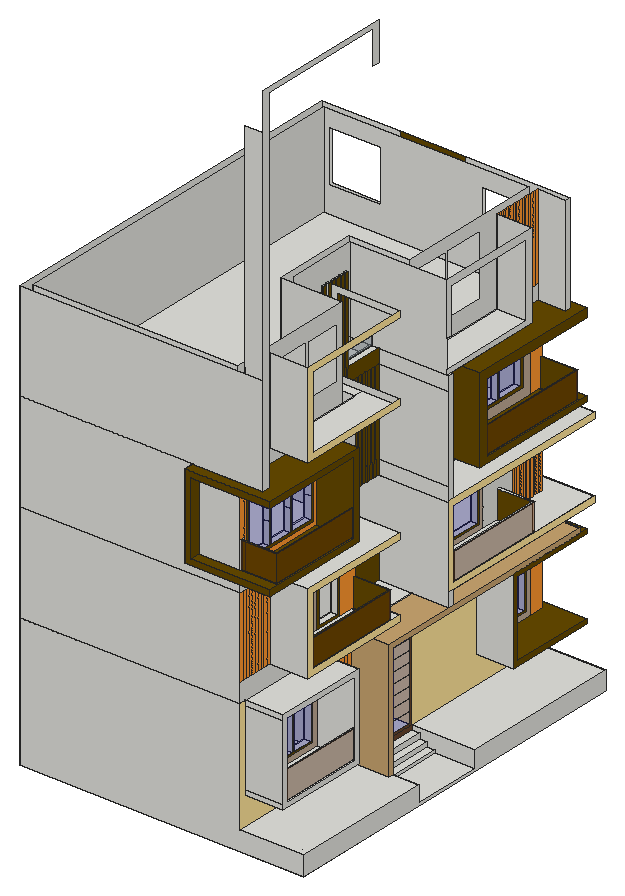
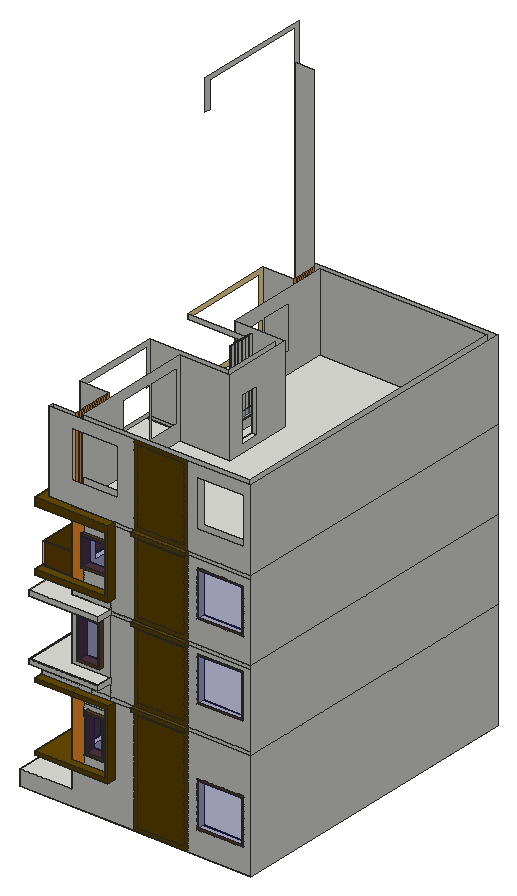
# SketchUp Ruby script. Lengths in inches.
U = 1.inch
M = Sketchup.active_model
def pt(a) = Geom::Point3d.new(a.map { |v| v * U })
def face(e, loops, mat)
  f = e.add_face(loops[0].map { |a| pt(a) })
  loops[1..].each { |l| e.add_face(l.map { |a| pt(a) }).erase! }
  f.material = f.back_material = mat if mat
  f
end
# faces: each face lists its corners as indices into pts; further lists are holes
def faces(e, pts, list, mat = nil) = list.each { |f| face(e, (f[0].is_a?(Array) ? f : [f]).map { |l| l.map { |i| pts[i] } }, mat) }
# xy, xz, yz: faces in a plane at the given z, y or x. An outline is a flat list of corners, or four numbers for a rectangle; further outlines are holes
def ring(l) = l.size == 4 ? [[l[0], l[1]], [l[2], l[1]], [l[2], l[3]], [l[0], l[3]]] : l.each_slice(2).to_a
def flat(e, list, mat, &to3) = list.each { |f| face(e, (f[0].is_a?(Array) ? f : [f]).map { |l| ring(l).map { |u, v| to3.(u, v) } }, mat) }
def xy(e, z, list, mat = nil) = flat(e, list, mat) { |x, y| [x, y, z] }
def xz(e, y, list, mat = nil) = flat(e, list, mat) { |x, z| [x, y, z] }
def yz(e, x, list, mat = nil) = flat(e, list, mat) { |y, z| [x, y, z] }
def lines(e, pts, list) = list.each { |a, b| e.add_line(pt(pts[a]), pt(pts[b])) }
# prism: a flat outline (further loops are holes) pulled along v
def prism(e, loops, v, mat = nil)
  f = face(e, loops, mat); d = Geom::Vector3d.new(v.map { |x| x * U })
  f.pushpull(f.normal.samedirection?(d) ? d.length : -d.length)
end
def box(e, o, s, mat = nil) = prism(e, [[o, [o[0] + s[0], o[1], o[2]], [o[0] + s[0], o[1] + s[1], o[2]], [o[0], o[1] + s[1], o[2]]]], [0, 0, s[2]], mat)
def at(x, y, z, deg = 0) = Geom::Transformation.translation(pt([x, y, z])) * Geom::Transformation.rotation(ORIGIN, Z_AXIS, deg.degrees)
def axes(o, x, y, z) = Geom::Transformation.new([*x, 0, *y, 0, *z, 0, *pt(o).to_a, 1])
def part(name) = M.definitions.add(name)
# library, detail: a bought-in or finely detailed component or shape, given as its bounding box
def library(name, o, s) = part(name).tap { |d| box(d.entities, o, s) }
def detail(e, o, s) = box(e.add_group.entities, o, s)
def put(e, d, t, mat = nil) = e.add_instance(d, t).tap { |i| i.material = mat if mat }
def group(e, t, mat = nil) = e.add_group.tap { |g| g.transformation = t; g.material = mat if mat }.entities
root = M.entities
M.materials.add("C04_Amber_Sunshine").color = [255, 152, 49]
M.materials.add("D02_Buttercup_Glow").color = [255, 229, 155]
M.materials.add("D08_Bronzed_Mustard").color = [102, 74, 0]
M.materials.add("Glass_Basic_01").color = [161, 173, 186]
M.materials["Glass_Basic_01"].alpha = 0.25
M.materials.add("Glass_Sky Reflection_01").color = [130, 55, 3]
M.materials["Glass_Sky Reflection_01"].alpha = 0.25
M.materials.add("Glass_Sky Reflection_1").color = [0, 2, 183]
M.materials["Glass_Sky Reflection_1"].alpha = 0.25
M.materials.add("Plywood_08_1K").color = [202, 166, 113]
M.materials.add("ThomThom - Complexion1").color = [190, 169, 148]
M.materials.add("Wood_Veneer_15_1K").color = [103, 69, 45]
xy(root,0,[[0,12,360,492]])
xy(root,3,[[309,195,360,285]])
xy(root,6,[[299,195,309,285]])
xy(root,12,[[289,195,299,285]])
xy(root,18,[[279,195,289,285]])
xy(root,24,[[279,12,360,12,360,195,327,195,327,189,279,189],[9,21,270,189],[9,195,279,285],[279,285,360,492],[9,291,270,483]])
xy(root,39,[[15,483,81,492]])
xy(root,60,[[279,21,327,141]])
xy(root,60,[[279,387,279,492,213,492,213,504,327,504,327,387]],"D08_Bronzed_Mustard")
xy(root,66,[[279,27,322.5,135],[322.5,27,324,135],[325.5,27,327,135]])
xy(root,66,[[279,393,327,393,327,504,219,504,219,492,279,492]],"D08_Bronzed_Mustard")
xy(root,75,[[270,36,279,66],[270,68,279,96],[270,98,279,126],[270,402,279,433.5],[270,435.5,279,465]])
xy(root,84,[[225,492,255,498]],"Wood_Veneer_15_1K")
xy(root,87,[[228,483,252,498]],"Wood_Veneer_15_1K")
xy(root,102,[[324,27,325.5,135]])
xy(root,105,[[15,483,81,492]])
xy(root,141,[[228,483,252,498]],"Wood_Veneer_15_1K")
xy(root,144,[[225,492,255,498]],"Wood_Veneer_15_1K")
xy(root,153,[[270,36,279,66],[270,68,279,96],[270,98,279,126],[270,402,279,433.5],[270,435.5,279,465]])
xy(root,162,[[279,27,327,135]])
xy(root,162,[[279,393,279,492,219,492,219,504,327,504,327,393]],"D08_Bronzed_Mustard")
xy(root,168,[[0,12,270,21],[0,21,9,492],[9,21,270,189],[279,21,327,141],[9,189,270,195],
  [270,195,279,285],[9,285,270,291],[270,285,279,285,279,387,327,387,327,492,270,492],[9,291,270,483],[9,483,270,492]])
xy(root,168,[[9,195,270,285]],"D02_Buttercup_Glow")
xy(root,168,[[99,492,183,498],[213,492,270,504],[270,492,327,504]],"D08_Bronzed_Mustard")
xy(root,168,[[279,195,327,387]],"Plywood_08_1K")
xy(root,174,[[9,21,270,186],[9,195,192,285],[201,195,234,285],[237,195,279,285],[9,294,270,483]])
xy(root,174,[[99,492,183,498]],"D08_Bronzed_Mustard")
xy(root,174,[[279,189,327,285],[279,291,327,492]],"Plywood_08_1K")
xy(root,177,[[192,240,201,270]])
xy(root,192,[[279,60,279,195,237,195,237,207.17,327,207.17,327,60],[234,195,237,205.43],[279,291,279,492,219,492,219,516,327,516,327,291]])
xy(root,198,[[279,67.85,322.5,67.85,322.5,70.5,283.5,70.5,283.5,190.5,279,190.5],[322.5,67.85,324,67.85,324,192,279,192,279,190.5,322.5,190.5],[283.5,70.5,322.5,190.5],[279,291,324,420]])
xy(root,199.85,[[325.5,67.85,327,67.85,327,195,279,195,279,193.5,325.5,193.5],[243,195,327,207.17],[325.5,291,327,423],[325.5,423,327,423,327,516,219,516,219,492,220.5,492,220.5,514.5,325.5,514.5],[279,423,325.5,423,325.5,514.5,220.5,514.5,220.5,492,279,492]])
xy(root,201,[[270,138,279,168]])
xy(root,207,[[270,300,279,345],[270,347,279,390]])
xy(root,210,[[231,492,267,498]])
xy(root,210,[[234,209,237,212.5],[234,216,237,219.5],[234,223,237,226.5],[234,230,237,233.5],[234,237,237,285]],"D08_Bronzed_Mustard")
xy(root,213,[[234,483,264,498]],"Wood_Veneer_15_1K")
xy(root,213.96,[[15,483,81,492]])
xy(root,234,[[324,67.85,325.5,67.85,325.5,193.5,279,193.5,279,192,324,192],[324,291,325.5,291,325.5,423,279,423,279,420,324,420]])
xy(root,255,[[192,240,201,270]])
xy(root,273,[[234,483,264,498]],"Wood_Veneer_15_1K")
xy(root,276,[[231,492,267,498]],"Wood_Veneer_15_1K")
xy(root,279,[[270,138,279,168],[270,300,279,345],[270,347,279,390]])
xy(root,279.96,[[15,483,81,492]])
xy(root,286.15,[[279,67.85,279,195,243,195,243,207.17,327,207.17,327,67.85]])
xy(root,288,[[279,291,279,492,219,492,219,516,327,516,327,291]])
xy(root,288,[[99,492,183,498]],"D08_Bronzed_Mustard")
xy(root,294,[[0,12,279,21],[0,21,9,492],[9,21,270,186],[270,21,279,195],[279,60,327,60,327,207.17,237,207.17,237,195,279,195],
  [9,186,270,186,270,195,201,195,201,285,192,285,192,195,9,195],[9,195,192,285],[201,195,201,285,237,285,237,237,234,237,234,195],[234,195,237,205.43],[234,209,237,212.5],
  [234,216,237,219.5],[234,223,237,226.5],[234,230,237,233.5],[9,285,192,294],[9,294,192,483],
  [192,294,270,483],[270,294,279,483],[9,483,192,492],[192,483,279,492]])
xy(root,294,[[99,492,183,498]],"D08_Bronzed_Mustard")
xy(root,295.85,[[279,291,327,291,327,516,219,516,219,492,279,492]])
xy(root,300,[[9,21,270,21,270,186,192,186,192,294,270,294,270,483,9,483],[201,195,226.5,285]])
xy(root,312,[[226.5,195,228,285],[229.5,195,237,195,237,246.5,234,246.5,234,285,229.5,285],[192,240,201,270],[234,250,237,253.5],[234,257,237,260.5],
  [234,264,237,267.5],[234,271,237,274.5],[234,278,237,281.5]])
xy(root,312,[[219,0,219,12,279,12,279,141,327,141,327,0],[279,333,279,492,213,492,213,504,327,504,327,333]],"D08_Bronzed_Mustard")
xy(root,318,[[279,15,324,15,324,133.15,322.5,133.15,322.5,16.5,279,16.5],[279,16.5,322.5,133.15],[279,345,322.5,487.5],[322.5,345,324,345,324,489,279,489,279,487.5,322.5,487.5]],"D08_Bronzed_Mustard")
xy(root,319.85,[[226.85,0,327,12],[279,12,327,12,327,133.15,325.5,133.15,325.5,13.5,279,13.5],[325.5,345,327,345,327,492,279,492,279,490.5,325.5,490.5],[219,492,327,504]],"D08_Bronzed_Mustard")
xy(root,324,[[228,195,229.5,285]],"Glass_Basic_01")
xy(root,327,[[270,27,279,60],[270,62,279,93],[270,95,279,126]])
xy(root,333,[[270,354,279,386.99],[270,389,279,421.99],[270,424,279,459],[15,483,81,492]])
xy(root,342,[[219,492,261,498]])
xy(root,345,[[222,483,258,498]],"Wood_Veneer_15_1K")
xy(root,354,[[279,13.5,325.5,13.5,325.5,133.15,324,133.15,324,15,279,15],[324,345,325.5,345,325.5,490.5,279,490.5,279,489,324,489]],"D08_Bronzed_Mustard")
xy(root,381,[[192,240,201,270]])
xy(root,387,[[222,483,258,498]],"Wood_Veneer_15_1K")
xy(root,390,[[219,492,261,498]],"Wood_Veneer_15_1K")
xy(root,399,[[270,354,279,386.99],[270,389,279,421.99],[270,424,279,459],[15,483,81,492]])
xy(root,405,[[270,27,279,60],[270,62,279,93],[270,95,279,126]])
xy(root,408,[[279,345,279,492,219,492,219,504,327,504,327,345]],"D08_Bronzed_Mustard")
xy(root,412.15,[[226.85,0,279,12],[279,0,327,133.15]],"D08_Bronzed_Mustard")
xy(root,414,[[99,492,183,498]],"D08_Bronzed_Mustard")
xy(root,420,[[0,12,270,21],[0,21,9,492],[9,21,9,483,192,483,192,186,270,186,270,21],[201,195,201,285,234,285,234,281.5,237,281.5,237,278,234,278,234,274.5,237,274.5,237,271,234,271,234,267.5,237,267.5,237,264,234,264,234,260.5,237,260.5,237,257,234,257,234,253.5,237,253.5,237,250,234,250,234,246.5,237,246.5,237,195],[192,294,270,483],
  [9,483,192,492],[192,483,279,492]])
xy(root,420,[[219,0,327,0,327,141,279,141,279,21,309,21,309,12,219,12],[279,333,327,333,327,504,213,504,213,492,315,492,315,484.8,279,484.8],[99,492,183,498]],"D08_Bronzed_Mustard")
xy(root,426,[[9,21,270,21,270,186,192,186,192,294,270,294,270,483,9,483],[201,195,226.5,285]])
xy(root,438,[[279,60,327,207.17],[226.5,195,228,285],[229.5,195,237,195,237,198.5,234,198.5,234,237,237,237,237,285,229.5,285],[240,195,279,207.17],[234,202,237,205.5],
  [234,209,237,212.5],[234,216,237,219.5],[234,223,237,226.5],[234,230,237,233.5],[192,240,201,270],
  [324,285,327,291],[279,291,324,420]])
xz(root,0,[[219,312,327,312,327,319.85,226.85,319.85,226.85,412.15,327,412.15,327,420,219,420]],"D08_Bronzed_Mustard")
xz(root,12,[[0,0,360,0,360,24,279,24,279,168,0,168],[0,168,279,294],[0,294,279,294,279,312,219,312,219,420,0,420],[226.85,319.85,279,412.15],[0,420,309,546]])
xz(root,13.5,[[279,319.85,325.5,354]],"Glass_Sky Reflection_01")
xz(root,15,[[279,318,283.5,354],[283.5,318,324,354]],"D08_Bronzed_Mustard")
xz(root,21,[[9,24,270,168],[279,60,327,66],[279,66,327,162],[279,162,327,168],[9,174,270,294],
  [9,300,270,420],[279,420,309,822],[9,426,270,546]])
xz(root,27,[[279,66,279,162,327,162,327,66,325.5,66,325.5,102,324,102,324,66],[270,327,279,354],[270,354,279,405]])
xz(root,36,[[270,75,279,153]])
xz(root,60,[[279,192,327,294],[270,327,279,354],[270,354,279,405],[279,438,327,546]])
xz(root,62,[[270,327,279,354],[270,354,279,405]])
xz(root,66,[[270,75,279,153]])
xz(root,67.85,[[279,198,279,286.15,327,286.15,327,199.85,325.5,199.85,325.5,234,324,234,324,198]])
xz(root,68,[[270,75,279,153]])
xz(root,93,[[270,327,279,354],[270,354,279,405]])
xz(root,95,[[270,327,279,354],[270,354,279,405]])
xz(root,96,[[270,75,279,153]])
xz(root,98,[[270,75,279,153]])
xz(root,126,[[270,75,279,153],[270,327,279,354],[270,354,279,405]])
xz(root,133.15,[[279,318,324,318,324,354,325.5,354,325.5,319.85,327,319.85,327,412.15,279,412.15]],"D08_Bronzed_Mustard")
xz(root,135,[[279,66,324,66,324,102,325.5,102,325.5,66,327,66,327,162,279,162]])
xz(root,138,[[270,201,279,279]])
xz(root,141,[[279,60,327,168]])
xz(root,141,[[279,312,327,420]],"D08_Bronzed_Mustard")
xz(root,168,[[270,201,279,279]])
xz(root,186,[[9,174,270,294],[192,300,270,420],[192,426,270,546]])
xz(root,189,[[9,24,270,168]])
xz(root,189,[[279,24,327,174]],"Plywood_08_1K")
xz(root,192,[[279,198,324,234]],"D08_Bronzed_Mustard")
xz(root,193.5,[[279,199.85,325.5,234]],"Glass_Sky Reflection_01")
xz(root,195,[[9,174,192,294],[201,174,201,294,237,294,237,192,234,192,234,174],[234,174,237,192],[237,174,279,192],[237,294,237,312,229.5,312,229.5,324,228,324,228,312,201,312,201,420,237,420,237,438,279,438,279,294],
  [201,300,226.5,312],[201,426,226.5,438],[201,438,228,444],[229.5,438,240,444]])
xz(root,195,[[243,199.85,279,286.15]],"C04_Amber_Sunshine")
xz(root,195,[[9,24,279,168]],"D02_Buttercup_Glow")
xz(root,195,[[309,3,309,6,299,6,299,12,289,12,289,18,279,18,279,168,327,168,327,24,360,24,360,3]],"Plywood_08_1K")
xz(root,198.5,[[234,438,237,546]])
xz(root,202,[[234,438,237,546]],"D08_Bronzed_Mustard")
xz(root,205.43,[[234,192,237,294]])
xz(root,205.5,[[234,438,237,546]])
xz(root,207.17,[[237,192,237,294,327,294,327,286.15,243,286.15,243,199.85,327,199.85,327,192],[240,438,240,546,327,546,327,538.15,246,538.15,246,445.85,327,445.85,327,438]])
xz(root,209,[[234,210,237,294],[234,438,237,546]],"D08_Bronzed_Mustard")
xz(root,212.5,[[234,210,237,294],[234,438,237,546]],"D08_Bronzed_Mustard")
xz(root,216,[[234,210,237,294],[234,438,237,546]],"D08_Bronzed_Mustard")
xz(root,219.5,[[234,210,237,294],[234,438,237,546]],"D08_Bronzed_Mustard")
xz(root,223,[[234,210,237,294],[234,438,237,546]],"D08_Bronzed_Mustard")
xz(root,226.5,[[234,210,237,294],[234,438,237,546]],"D08_Bronzed_Mustard")
xz(root,230,[[234,210,237,294],[234,438,237,546]],"D08_Bronzed_Mustard")
xz(root,233.5,[[234,210,237,294],[234,438,237,546]],"D08_Bronzed_Mustard")
xz(root,237,[[234,210,237,294],[234,438,237,546]],"D08_Bronzed_Mustard")
xz(root,240,[[192,177,201,255],[192,312,201,381],[192,438,201,507]])
xz(root,246.5,[[234,312,237,420]],"D08_Bronzed_Mustard")
xz(root,250,[[234,312,237,420]],"D08_Bronzed_Mustard")
xz(root,253.5,[[234,312,237,420]],"D08_Bronzed_Mustard")
xz(root,257,[[234,312,237,420]],"D08_Bronzed_Mustard")
xz(root,260.5,[[234,312,237,420]],"D08_Bronzed_Mustard")
xz(root,264,[[234,312,237,420]],"D08_Bronzed_Mustard")
xz(root,267.5,[[234,312,237,420]],"D08_Bronzed_Mustard")
xz(root,270,[[192,177,201,255],[192,312,201,381],[192,438,201,507]])
xz(root,271,[[234,312,237,420]],"D08_Bronzed_Mustard")
xz(root,274.5,[[234,312,237,420]],"D08_Bronzed_Mustard")
xz(root,278,[[234,312,237,420]],"D08_Bronzed_Mustard")
xz(root,281.5,[[234,312,237,420]],"D08_Bronzed_Mustard")
xz(root,285,[[309,3,360,3,360,24,279,24,279,18,289,18,289,12,299,12,299,6,309,6],[9,174,192,294],[192,174,201,294],[201,174,234,174,234,210,237,210,237,174,327,174,327,294,201,294],[237,294,327,312],
  [201,300,226.5,312],[201,312,228,312,228,324,229.5,324,229.5,312,234,312,234,420,201,420],[237,312,327,420],[237,420,327,438],[201,426,226.5,438],
  [201,438,228,438,228,450,229.5,450,229.5,438,324,438,324,546,201,546]])
xz(root,285,[[9,24,279,168]],"D02_Buttercup_Glow")
xz(root,291,[[9,24,270,168],[279,174,327,192],[279,198,279,288,327,288,327,199.85,325.5,199.85,325.5,234,324,234,324,198],[279,295.85,327,438]])
xz(root,294,[[9,174,270,294],[192,300,270,420],[192,426,270,546]])
xz(root,300,[[270,207,279,279]])
xz(root,333,[[279,312,327,420]],"D08_Bronzed_Mustard")
xz(root,345,[[270,207,279,279]])
xz(root,345,[[279,318,279,408,327,408,327,319.85,325.5,319.85,325.5,354,324,354,324,318]],"D08_Bronzed_Mustard")
xz(root,347,[[270,207,279,279]])
xz(root,354,[[270,333,279,399]])
xz(root,386.99,[[270,333,279,399]])
xz(root,387,[[279,60,327,168]])
xz(root,389,[[270,333,279,399]])
xz(root,390,[[270,207,279,279]])
xz(root,393,[[279,66,327,162]],"D08_Bronzed_Mustard")
xz(root,402,[[270,75,279,153]])
xz(root,420,[[279,438,324,546]])
xz(root,420,[[279,198,324,234]],"D08_Bronzed_Mustard")
xz(root,421.99,[[270,333,279,399]])
xz(root,423,[[279,199.85,325.5,234]],"Glass_Sky Reflection_01")
xz(root,424,[[270,333,279,399]])
xz(root,433.5,[[270,75,279,153]])
xz(root,435.5,[[270,75,279,153]])
xz(root,459,[[270,333,279,399]])
xz(root,465,[[270,75,279,153]])
xz(root,483,[[[9,24,270,168],[15,39,81,105],[228,87,252,141]],[[9,174,249,174,249,213,234,213,234,273,249,273,249,294,9,294],[15,213.96,81,279.96]],[249,174,270,174,270,294,249,294,249,273,264,273,264,213,249,213],[[9,300,270,420],[15,333,81,399],[222,345,258,387]],[[9,426,270,426,270,459,210,459,210,525,270,525,270,546,9,546],[15,459,81,525]]])
xz(root,484.8,[[279,420,315,546]])
xz(root,489,[[279,318,324,354]],"D08_Bronzed_Mustard")
xz(root,490.5,[[279,319.85,325.5,354]],"Glass_Sky Reflection_01")
xz(root,492,[[[0,0,99,168],[12,36,84,108]],[183,0,183,168,213,168,213,60,279,60,279,24,360,24,360,0],[219,66,261,78],[[219,78,261,150],[225,84,255,144]],[219,150,261,162],
  [0,168,99,174],[183,168,219,174],[219,168,249,174],[249,168,327,174],[[0,174,99,288],[12,210.96,84,282.96]],
  [183,174,219,288],[219,174,279,192],[[219,199.85,279,288],[231,210,267,276]],[0,288,99,294],[183,288,219,294],
  [[0,294,99,414],[12,330,84,402]],[183,294,183,414,213,414,213,312,219,312,219,294],[219,294,279,295.85],[219,295.85,279,312],[219,319.85,261,342],
  [219,390,261,408],[0,414,99,420],[183,414,213,420],[[0,420,99,546],[12,456,84,528]],[[183,420,315,546],[207,456,279,528]]])
xz(root,492,[[261,66,279,162],[261,319.85,279,408]],"C04_Amber_Sunshine")
xz(root,492,[[[99,0,183,168],[105,6,177,162]],[105,6,177,162],[[99,174,183,288],[105,180,177,282]],[105,180,177,282],[[99,294,183,414],[105,300,177,408]],
  [105,300,177,408],[[99,420,183,546],[105,426,177,540]],[105,426,177,540]],"D08_Bronzed_Mustard")
xz(root,492,[[15,39,81,105],[15,213.96,81,279.96],[15,333,81,399]],"Glass_Sky Reflection_1")
xz(root,492,[[[12,36,84,108],[15,39,81,105]],[[12,210.96,84,282.96],[15,213.96,81,279.96]],[[12,330,84,402],[15,333,81,399]]],"Wood_Veneer_15_1K")
xz(root,498,[[99,168,183,174],[99,288,183,294],[99,414,183,420]],"D08_Bronzed_Mustard")
xz(root,498,[[228,87,252,141],[234,213,264,273],[222,345,258,387]],"Glass_Sky Reflection_1")
xz(root,498,[[[225,84,255,144],[228,87,252,141]],[[231,210,267,276],[234,213,264,273]],[[219,342,261,390],[222,345,258,387]]],"Wood_Veneer_15_1K")
xz(root,504,[[213,60,213,168,327,168,327,162,219,162,219,66,327,66,327,60],[213,312,213,420,327,420,327,408,219,408,219,319.85,327,319.85,327,312]],"D08_Bronzed_Mustard")
xz(root,516,[[219,192,327,199.85],[219,288,327,295.85]])
yz(root,0,[[12,0,492,168],[12,168,492,294],[12,294,492,420],[12,420,492,546]])
yz(root,9,[[21,24,189,168],[189,24,195,168],[285,24,291,168],[291,24,483,168],[21,174,186,294],
  [195,174,285,294],[294,174,483,294],[21,300,483,420],[21,426,483,546]])
yz(root,9,[[195,24,285,168]],"D02_Buttercup_Glow")
yz(root,15,[[483,39,492,105],[483,213.96,492,279.96],[483,333,492,399]])
yz(root,81,[[483,39,492,105],[483,213.96,492,279.96],[483,333,492,399]])
yz(root,99,[[492,168,498,174],[492,288,498,294],[492,414,498,420]],"D08_Bronzed_Mustard")
yz(root,183,[[492,168,498,174],[492,288,498,294],[492,414,498,420]],"D08_Bronzed_Mustard")
yz(root,192,[[[195,174,285,294],[240,177,270,255]],[[186,300,294,420],[240,312,270,381]],[[186,426,294,546],[240,438,270,507]]])
yz(root,201,[[195,174,237,174,237,258,273,258,273,174,285,174,285,294,195,294],[195,300,237,312],[237,300,273,300,273,312,270,312,270,303,240,303,240,312,237,312],[273,300,285,312],[240,303,270,312],
  [195,312,237,312,237,384,273,384,273,312,285,312,285,420,195,420],[195,426,237,438],[237,426,273,426,273,438,270,438,270,429,240,429,240,438,237,438],[273,426,285,438],[240,429,270,438],
  [195,438,237,438,237,510,273,510,273,438,285,438,285,546,195,546]])
yz(root,201,[[[237,174,273,258],[240,177,270,255]],[237,312,240,312,240,381,270,381,270,312,273,312,273,384,237,384],[237,438,240,438,240,507,270,507,270,438,273,438,273,510,237,510]],"D08_Bronzed_Mustard")
yz(root,213,[[492,60,504,168],[492,312,504,420]],"D08_Bronzed_Mustard")
yz(root,219,[[492,192,516,199.85],[492,288,516,295.85]])
yz(root,219,[[492,66,504,162],[0,312,12,318],[0,318,12,420],[492,319.85,504,319.85,504,408,492,408,492,390,498,390,498,342,492,342]],"D08_Bronzed_Mustard")
yz(root,222,[[483,345,498,387]],"Wood_Veneer_15_1K")
yz(root,225,[[492,84,498,144]])
yz(root,226.5,[[195,300,285,312],[195,426,285,438]])
yz(root,226.85,[[0,319.85,12,412.15]],"D08_Bronzed_Mustard")
yz(root,228,[[195,312,285,324],[195,438,285,450]],"Glass_Basic_01")
yz(root,228,[[483,87,498,141]],"Wood_Veneer_15_1K")
yz(root,229.5,[[195,312,285,324],[195,438,285,450]],"Glass_Basic_01")
yz(root,231,[[492,210,498,276]],"Wood_Veneer_15_1K")
yz(root,234,[[195,174,195,192,205.43,192,205.43,294,209,294,209,210,212.5,210,212.5,174],[212.5,174,212.5,294,216,294,216,210,219.5,210,219.5,174],[219.5,174,219.5,294,223,294,223,210,226.5,210,226.5,174],[226.5,174,230,294],[230,174,230,210,233.5,210,233.5,294,237,294,237,210,285,210,285,174],
  [246.5,312,250,420],[253.5,312,257,420],[260.5,312,264,420],[267.5,312,271,420],[274.5,312,278,420],
  [281.5,312,285,420],[198.5,438,202,546],[205.5,438,209,546],[212.5,438,216,546],[219.5,438,223,546],
  [226.5,438,230,546],[233.5,438,237,546]])
yz(root,234,[[483,213,498,273]],"Wood_Veneer_15_1K")
yz(root,237,[[195,192,205.43,294],[205.43,192,205.5,294],[205.5,192,207.17,294]])
yz(root,237,[[195,174,285,174,285,210,207.17,210,207.17,192,195,192],[207.17,210,209,210,209,312,205.5,312,205.5,294,207.17,294],[212.5,210,216,312],[219.5,210,223,312],[226.5,210,230,312],
  [233.5,210,237,312],[195,294,198.5,312],[198.5,294,202,312],[202,294,205.5,312],[209,294,212.5,312],
  [216,294,219.5,312],[223,294,226.5,312],[230,294,233.5,312],[237,294,246.5,312],[246.5,294,250,420],
  [250,294,253.5,312],[253.5,294,257,420],[257,294,260.5,312],[260.5,294,264,420],[264,294,267.5,312],
  [267.5,294,271,420],[271,294,274.5,312],[274.5,294,278,420],[278,294,281.5,312],[281.5,294,285,420],
  [195,420,198.5,438],[198.5,420,202,546],[202,420,205.5,438],[205.5,420,209,546],[209,420,212.5,438],
  [212.5,420,216,546],[216,420,219.5,438],[219.5,420,223,546],[223,420,226.5,438],[226.5,420,230,546],
  [230,420,233.5,438],[233.5,420,237,546],[237,420,285,438]],"D08_Bronzed_Mustard")
yz(root,240,[[195,438,207.17,444]])
yz(root,243,[[195,199.85,207.17,286.15]])
yz(root,252,[[483,87,498,141]],"Wood_Veneer_15_1K")
yz(root,255,[[492,84,498,144]],"Wood_Veneer_15_1K")
yz(root,258,[[483,345,498,387]],"Wood_Veneer_15_1K")
yz(root,261,[[492,342,498,390]],"Wood_Veneer_15_1K")
yz(root,264,[[483,213,498,273]],"Wood_Veneer_15_1K")
yz(root,267,[[492,210,498,276]],"Wood_Veneer_15_1K")
yz(root,270,[[[21,24,189,168],[36,75,66,153],[68,75,96,153],[98,75,126,153]],[[291,24,483,168],[402,75,433.5,153],[435.5,75,465,153]],[[21,174,186,294],[138,201,168,279]],[[294,174,483,294],[300,207,345,279],[347,207,390,279]],[[21,300,186,420],[27,327,60,405],[62,327,93,405],[95,327,126,405]],
  [[294,300,483,420],[424,333,459,399],[389,333,421.99,399],[354,333,386.99,399]],[[21,426,186,546],[81,459,129,525],[131,459,177,525]],[[294,426,483,546],[352.5,453,405,531],[300,453,350.5,531]]])
yz(root,279,[[12,168,189,168,189,174,195,174,195,192,12,192],[195,168,285,174],[291,174,492,192],[399,198,420,198,420,234,423,234,423,199.85,444,199.85,444,288,399,288],[12,294,195,294,195,438,21,438,21,420,141,420,141,312,12,312],
  [291,294,294,295.85],[294,294,483,295.85],[483,294,492,295.85],[291,295.85,492,295.85,492,312,333,312,333,420,484.8,420,484.8,438,291,438],[15,318,18,354],
  [12,319.85,13.5,354]])
yz(root,279,[[141,60,147,168],[147,60,153,168],[153,60,159,168],[159,60,165,168],[165,60,171,168],
  [171,60,177,168],[177,60,183,168],[183,60,189,168],[474,66,492,162],[12,192,16.8,294],
  [16.8,192,21.6,294],[21.6,192,26.4,294],[26.4,192,31.2,294],[31.2,192,36,294],[36,192,40.8,294],
  [40.8,192,45.6,294],[45.6,192,50.4,294],[50.4,192,55.2,294],[55.2,192,60,294],[171,198,192,198,192,234,193.5,234,193.5,199.85,195,199.85,195,286.15,171,286.15],
  [444,199.85,447,288],[447,199.85,450,288],[450,199.85,453,288],[453,199.85,456,288],[456,199.85,459,288],
  [459,199.85,462,288],[462,199.85,465,288],[465,199.85,468,288],[468,199.85,471,288],[471,199.85,474,288],
  [474,199.85,477,288],[477,199.85,480,288],[480,199.85,483,288],[483,199.85,486,288],[486,199.85,489,288],
  [489,199.85,492,288],[[18,318,133.15,412.15],[24,324,129,408]],[474,318,489,318,489,354,490.5,354,490.5,319.85,492,319.85,492,408,474,408],[12,354,18,412.15],[21,438,24.9,546],
  [24.9,438,28.8,546],[28.8,438,32.7,546],[32.7,438,36.6,546],[36.6,438,40.5,546],[40.5,438,44.4,546],
  [44.4,438,48.3,546],[48.3,438,52.2,546],[52.2,438,56.1,546],[56.1,438,60,546],[420,438,423.6,546],
  [423.6,438,427.2,546],[427.2,438,430.8,546],[430.8,438,434.4,546],[434.4,438,438,546],[438,438,441.6,546],
  [441.6,438,445.2,546],[445.2,438,448.8,546],[448.8,438,452.4,546],[452.4,438,456,546],[456,438,459.6,546],
  [459.6,438,463.2,546],[463.2,438,466.8,546],[466.8,438,470.4,546],[470.4,438,474,546],[474,438,477.6,546],
  [477.6,438,481.2,546],[481.2,438,484.8,546]],"C04_Amber_Sunshine")
yz(root,279,[[12,24,189,24,189,60,21,60,21,168,12,168],[285,24,492,24,492,60,387,60,387,168,285,168]],"D02_Buttercup_Glow")
yz(root,279,[[[33,72,129,156],[36,75,36,153,66,153,66,75,68,75,68,153,96,153,96,75,98,75,98,153,126,153,126,75]],[[399,72,468,156],[402,75,402,153,465,153,465,75,435.5,75,435.5,153,433.5,153,433.5,75]],[[135,198,171,282],[138,201,168,279]],[[297,204,393,282],[300,207,300,279,390,279,390,207,347,207,347,279,345,279,345,207]],[[24,324,129,408],[27,327,27,405,60,405,60,327,62,327,62,405,93,405,93,327,95,327,95,405,126,405,126,327]],
  [[351,330,462,402],[354,333,354,399,386.99,399,386.99,333,389,333,389,399,421.99,399,421.99,333,424,333,424,399,459,399,459,333]]],"D08_Bronzed_Mustard")
yz(root,279,[[198,27,237,40.8],[243,27,282,40.8],[198,40.8,237,54.6],[243,40.8,282,54.6],[198,54.6,237,68.4],
  [243,54.6,282,68.4],[198,68.4,237,82.2],[243,68.4,282,82.2],[36,75,66,153],[68,75,96,153],
  [98,75,126,153],[402,75,433.5,153],[435.5,75,465,153],[198,82.2,237,96],[243,82.2,282,96],
  [198,96,237,109.8],[243,96,282,109.8],[198,109.8,237,123.6],[243,109.8,282,123.6],[198,123.6,237,137.4],
  [243,123.6,282,137.4],[198,137.4,237,151.2],[243,137.4,282,151.2],[198,151.2,237,165],[243,151.2,282,165],
  [300,207,345,279],[347,207,390,279],[27,327,60,405],[62,327,93,405],[95,327,126,405],
  [354,333,386.99,399],[389,333,421.99,399],[424,333,459,399]],"Glass_Sky Reflection_1")
yz(root,279,[[[27,66,135,162],[33,72,129,156]],[[393,66,474,162],[399,72,468,156]],[67.85,198,135,198,135,282,171,282,171,286.15,67.85,286.15],[[291,198,399,288],[297,204,393,282]],[[345,318,474,408],[351,330,462,402]]],"ThomThom - Complexion1")
yz(root,279,[[195,18,285,24],[[195,24,240,168],[198,27,237,165]],[[240,24,285,168],[243,27,282,165]]],"Wood_Veneer_15_1K")
yz(root,289,[[195,12,285,18]])
yz(root,299,[[195,6,285,12]])
yz(root,309,[[195,3,285,6],[12,420,21,420,21,870,186,870,186,828,195,828,195,876,12,876]])
yz(root,315,[[484.8,420,492,546]])
yz(root,324,[[27,66,135,102],[67.85,198,70.5,234],[291,198,295.5,234],[295.5,198,420,234],[285,438,420,438,420,546,285,546,285,480,291,480,291,537,411,537,411,444,285,444]])
yz(root,324,[[70.5,198,192,234],[15,318,133.15,354],[345,318,489,354]],"D08_Bronzed_Mustard")
yz(root,325.5,[[27,66,135,102],[67.85,199.85,193.5,234],[291,199.85,423,234],[13.5,319.85,133.15,354],[345,319.85,490.5,354]],"Glass_Sky Reflection_01")
yz(root,327,[[[21,60,141,168],[27,66,135,162]],[285,174,291,192],[285,295.85,291,438]])
yz(root,327,[[60,192,207.17,192,207.17,199.85,67.85,199.85,67.85,286.15,207.17,286.15,207.17,294,60,294],[285,192,516,192,516,199.85,291,199.85,291,288,516,288,516,295.85,285,295.85],[60,438,207.17,438,207.17,445.85,67.85,445.85,67.85,538.15,207.17,538.15,207.17,546,60,546]],"D02_Buttercup_Glow")
yz(root,327,[[387,60,504,60,504,66,393,66,393,162,504,162,504,168,387,168],[0,312,141,312,141,420,0,420,0,412.15,133.15,412.15,133.15,319.85,0,319.85],[333,312,504,312,504,319.85,345,319.85,345,408,504,408,504,420,333,420]],"D08_Bronzed_Mustard")
yz(root,327,[[189,24,195,24,195,168,492,168,492,174,189,174]],"Plywood_08_1K")
yz(root,360,[[12,0,492,0,492,24,285,24,285,3,195,3,195,24,12,24]])
p = [[351,21,0],[351,21,24],[9,483,0],[9,483,24],[9,21,0],[9,21,24],
  [249,492,162],[249,492,168],[270,186,420],[279,186,420],[270,294,420],[279,294,420],
  [234,285,420],[237,285,420],[279,291,444],[279,291,438],[219,492,414],[213,492,414]]
lines(root,p,[[0,1],[2,3],[4,5],[6,7],[8,9],[10,11],[12,13],[14,15],[16,17]])
